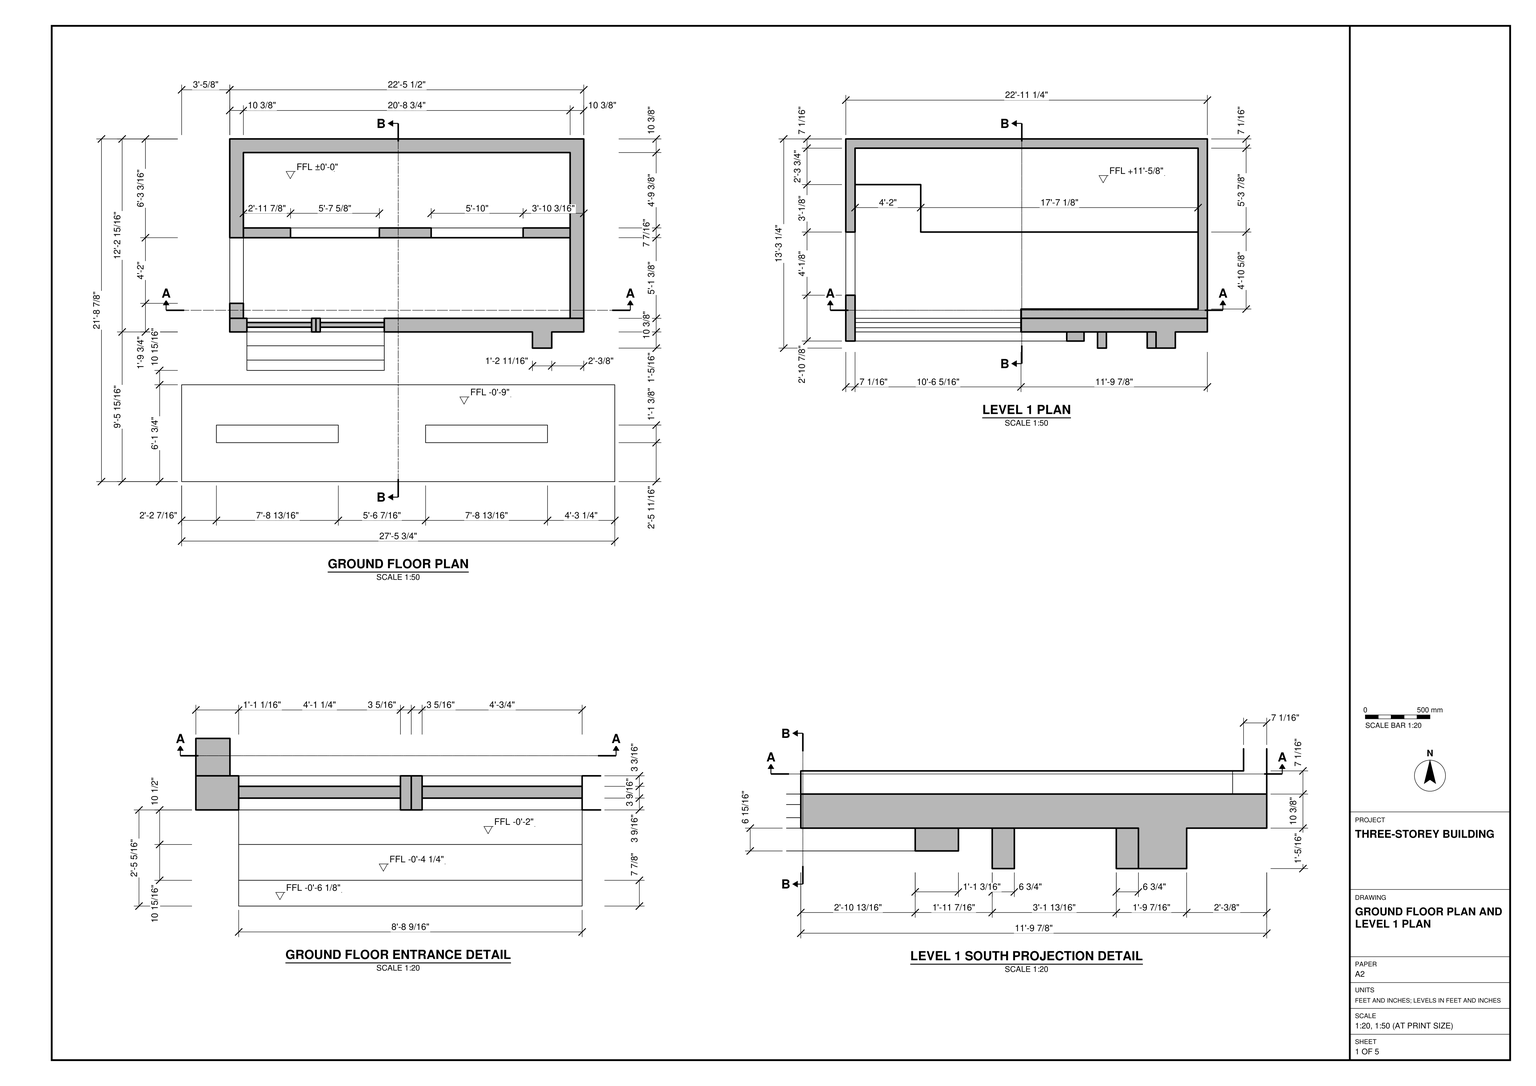
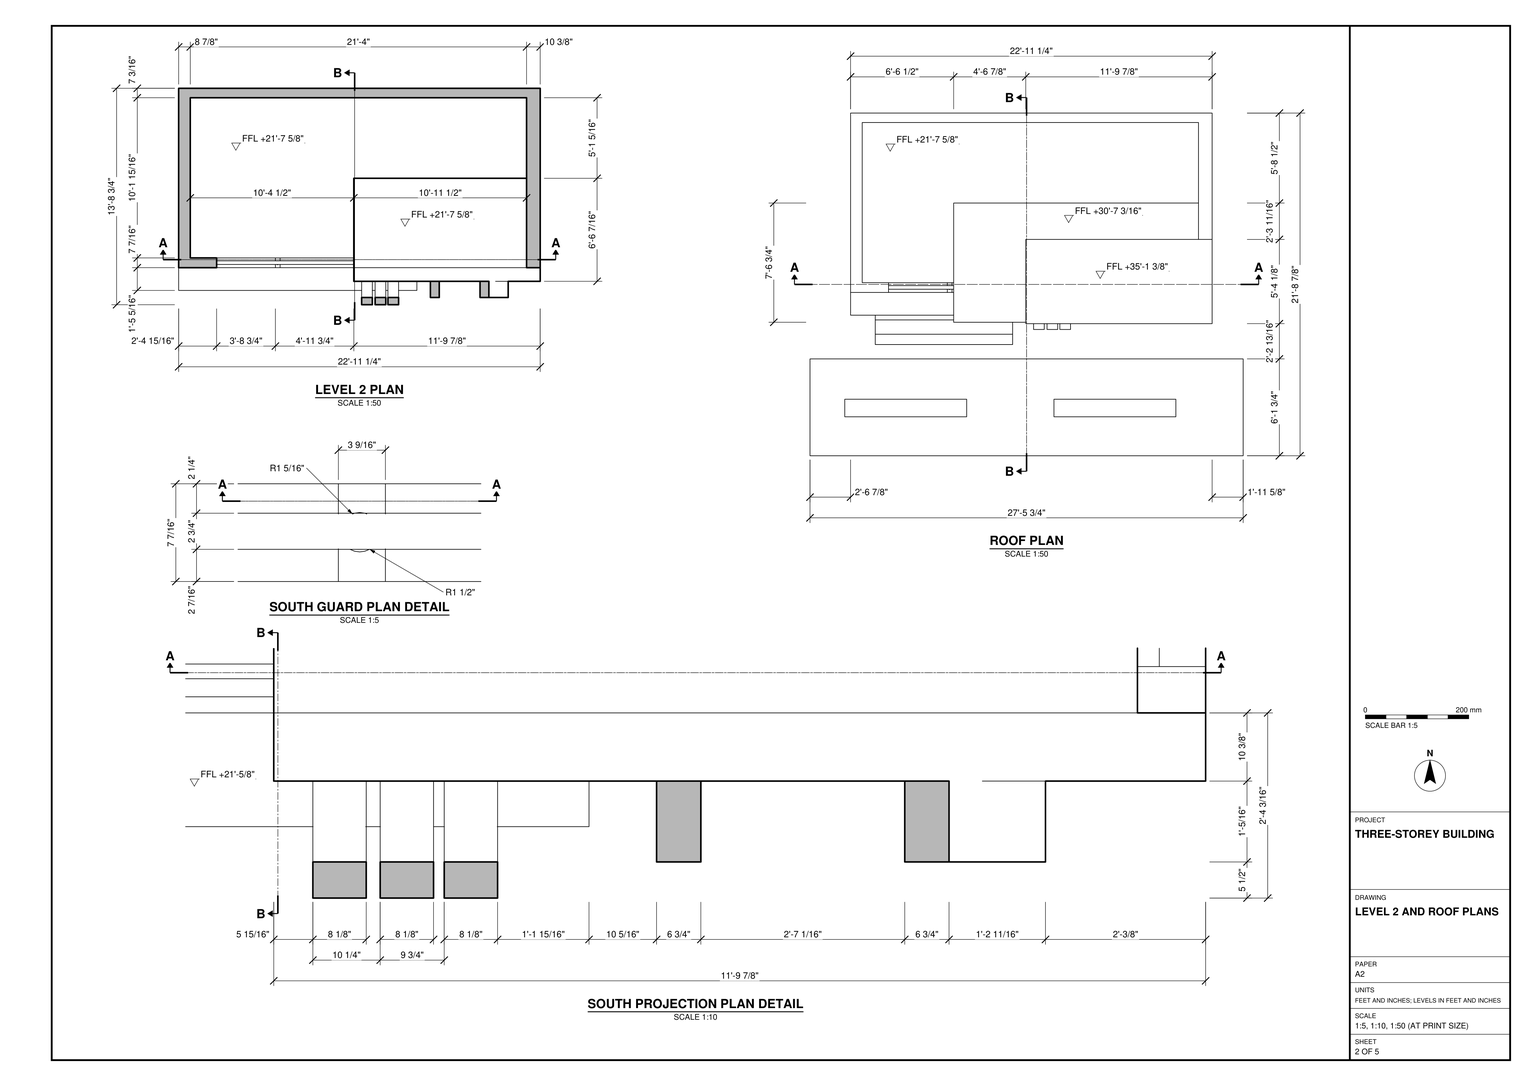
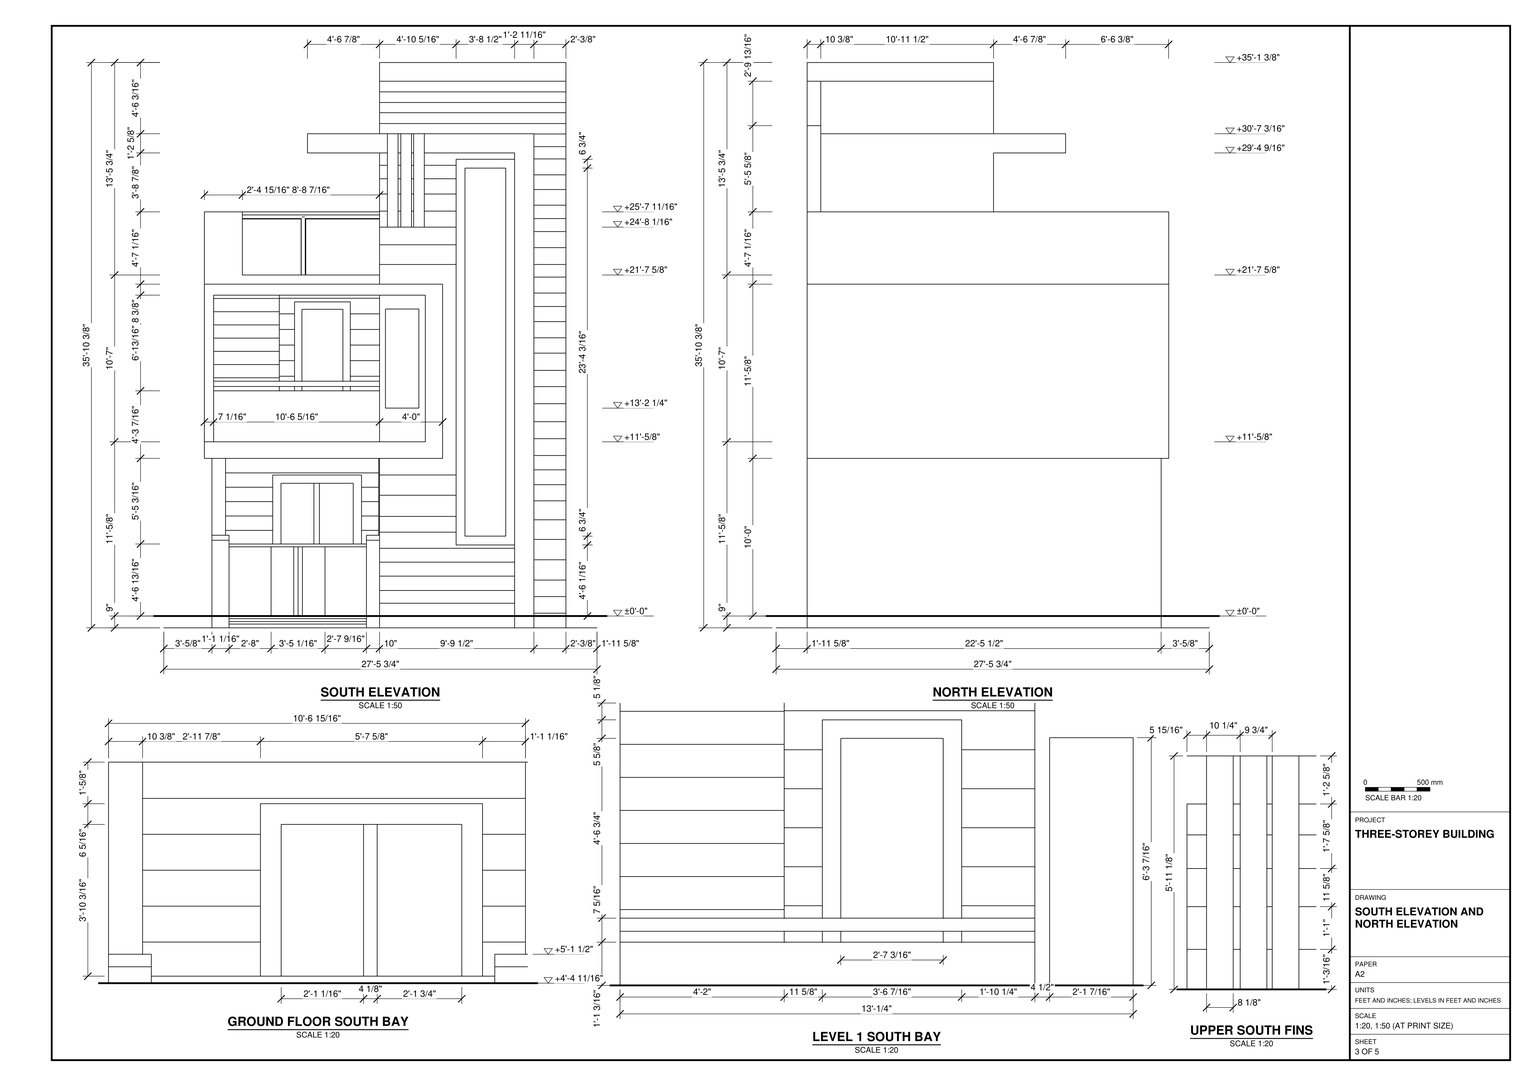
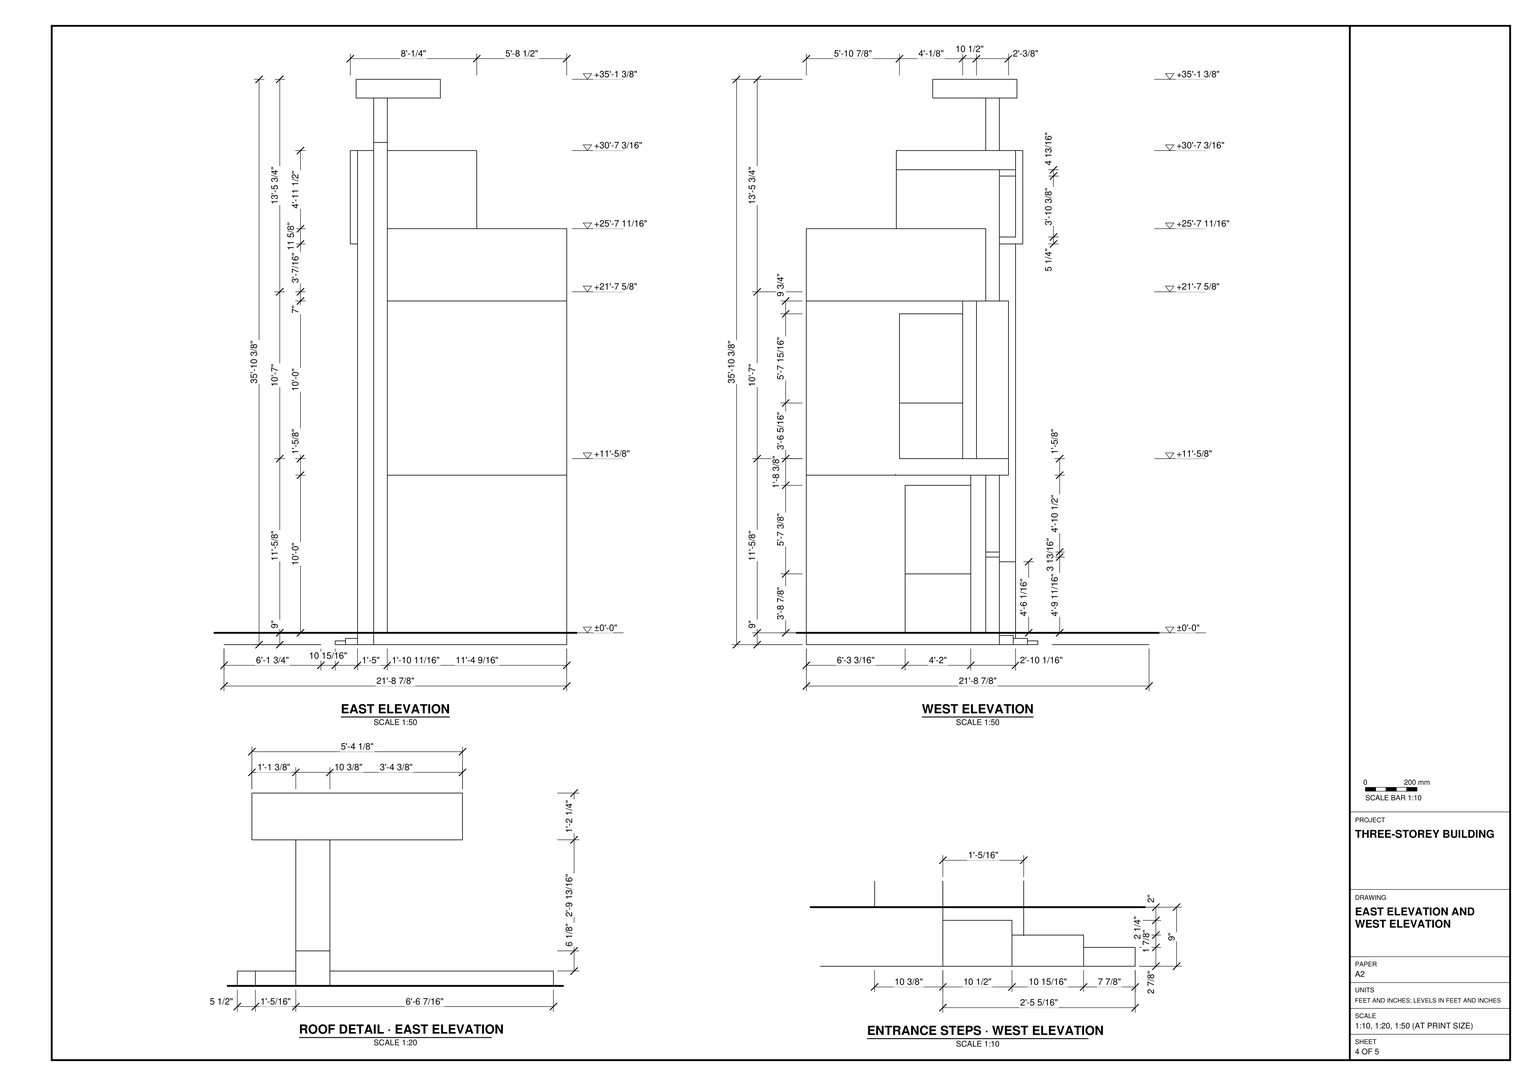
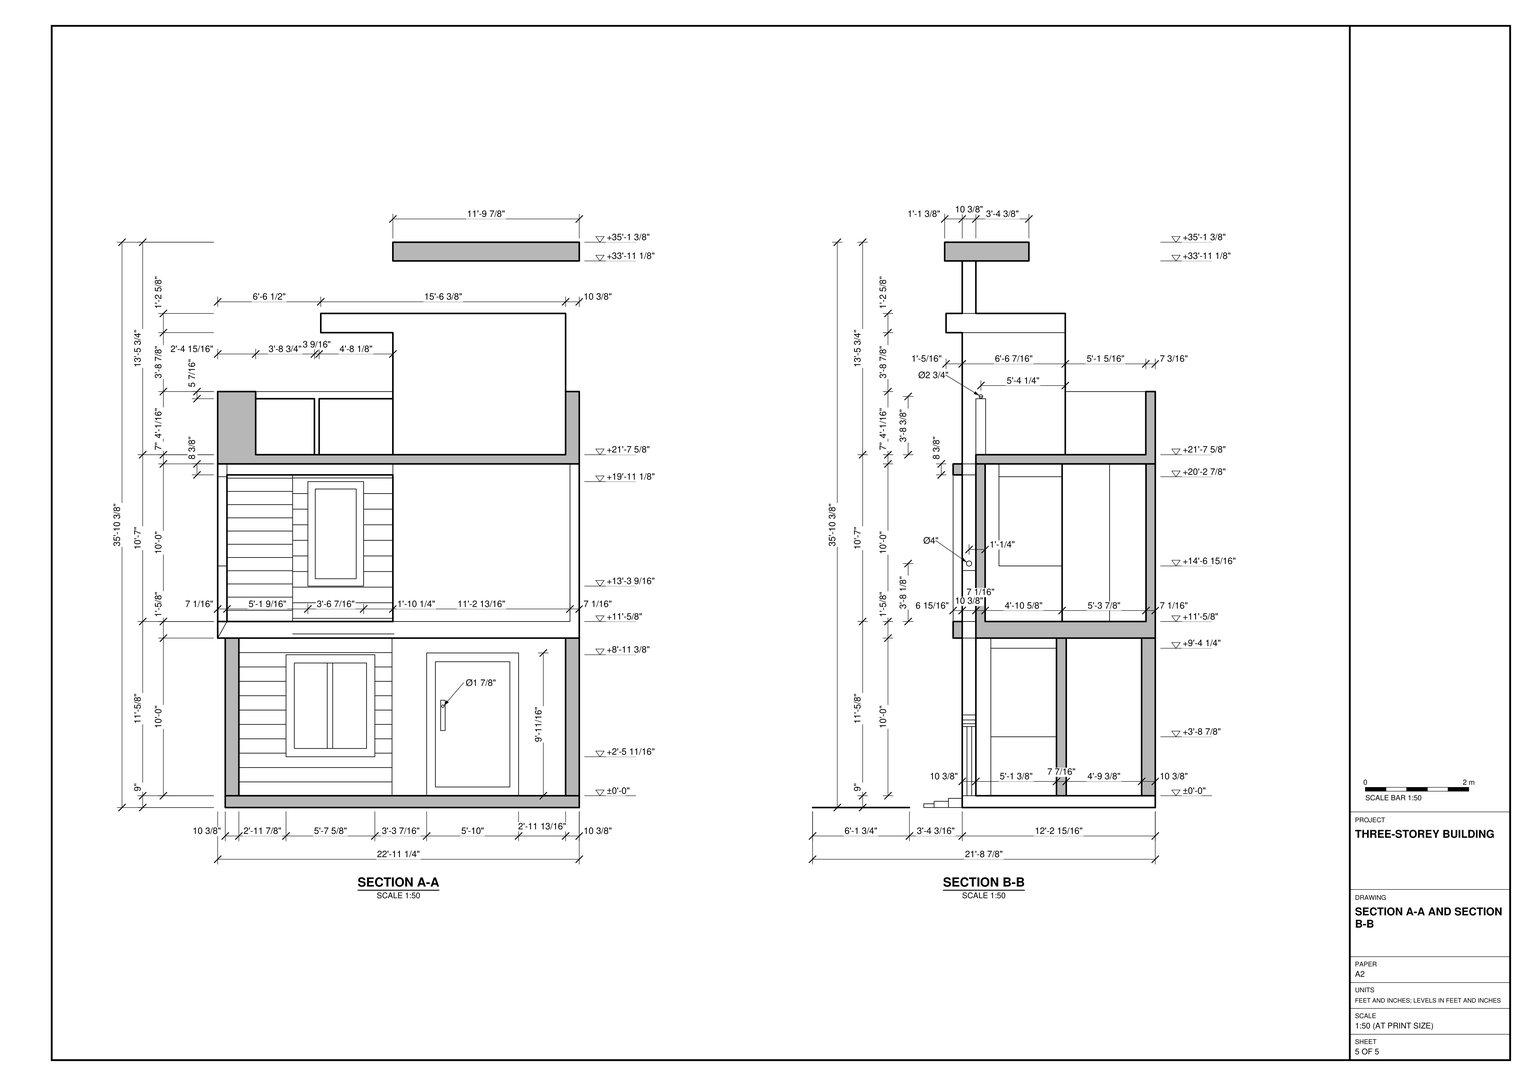
Build the three-storey building in SketchUp from task_files/diagram_01.pdf. Work in feet and inches. Set the ground floor at ±0'-0", Level 1 at +11'-5/8" and Level 2 at +21'-7 5/8". Including the ground strip in front of the entrance, the model must measure 27'-5 3/4" along X, 21'-8 7/8" along Y and 35'-10 3/8" along Z.

Follow the plan for each storey rather than repeating the ground-floor footprint. Model the floor slabs, walls and openings with the offsets and thicknesses drawn, including the 10 3/8" ground-floor side walls and the 7 1/16" Level 1 side walls. On the south side, build the entrance steps, the divided ground-floor opening and the projecting frame around the Level 1 bay. Use the enlarged details to place the guards, upper fins and tall framed panel. Match the horizontal divisions on the south face and the stepped outline of the flat roof to the elevations. Include the two narrow rectangular features on the front ground strip.

Keep walls, slabs and roof elements in separate groups or components. Keep each furniture or joinery piece shown separate, and use components for repeated parts. Any decor or loose items shown may be represented by suitable library components. Save one SketchUp model as output_files/three_storey_building_with_projecting_south_bays.skp.

# SketchUp Ruby script. Lengths in inches.
U = 1.inch
M = Sketchup.active_model
def pt(a) = Geom::Point3d.new(a.map { |v| v * U })
def face(e, loops, mat)
  f = e.add_face(loops[0].map { |a| pt(a) })
  loops[1..].each { |l| e.add_face(l.map { |a| pt(a) }).erase! }
  f.material = f.back_material = mat if mat
  f
end
# faces: each face lists its corners as indices into pts; further lists are holes
def faces(e, pts, list, mat = nil) = list.each { |f| face(e, (f[0].is_a?(Array) ? f : [f]).map { |l| l.map { |i| pts[i] } }, mat) }
# xy, xz, yz: faces in a plane at the given z, y or x. An outline is a flat list of corners, or four numbers for a rectangle; further outlines are holes
def ring(l) = l.size == 4 ? [[l[0], l[1]], [l[2], l[1]], [l[2], l[3]], [l[0], l[3]]] : l.each_slice(2).to_a
def flat(e, list, mat, &to3) = list.each { |f| face(e, (f[0].is_a?(Array) ? f : [f]).map { |l| ring(l).map { |u, v| to3.(u, v) } }, mat) }
def xy(e, z, list, mat = nil) = flat(e, list, mat) { |x, y| [x, y, z] }
def xz(e, y, list, mat = nil) = flat(e, list, mat) { |x, z| [x, y, z] }
def yz(e, x, list, mat = nil) = flat(e, list, mat) { |y, z| [x, y, z] }
def lines(e, pts, list) = list.each { |a, b| e.add_line(pt(pts[a]), pt(pts[b])) }
# prism: a flat outline (further loops are holes) pulled along v
def prism(e, loops, v, mat = nil)
  f = face(e, loops, mat); d = Geom::Vector3d.new(v.map { |x| x * U })
  f.pushpull(f.normal.samedirection?(d) ? d.length : -d.length)
end
def box(e, o, s, mat = nil) = prism(e, [[o, [o[0] + s[0], o[1], o[2]], [o[0] + s[0], o[1] + s[1], o[2]], [o[0], o[1] + s[1], o[2]]]], [0, 0, s[2]], mat)
def at(x, y, z, deg = 0) = Geom::Transformation.translation(pt([x, y, z])) * Geom::Transformation.rotation(ORIGIN, Z_AXIS, deg.degrees)
def axes(o, x, y, z) = Geom::Transformation.new([*x, 0, *y, 0, *z, 0, *pt(o).to_a, 1])
def part(name) = M.definitions.add(name)
# library, detail: a bought-in or finely detailed component or shape, given as its bounding box
def library(name, o, s) = part(name).tap { |d| box(d.entities, o, s) }
def detail(e, o, s) = box(e.add_group.entities, o, s)
def put(e, d, t, mat = nil) = e.add_instance(d, t).tap { |i| i.material = mat if mat }
def group(e, t, mat = nil) = e.add_group.tap { |g| g.transformation = t; g.material = mat if mat }.entities
root = M.entities
M.materials.add("[0012_Bisque]").color = [255, 228, 196]
M.materials.add("[0061_OliveDrab]").color = [96, 127, 31]
M.materials.add("[Asphalt New]").color = [67, 60, 62]
M.materials.add("[Carpet Diamond Yellow]").color = [226, 217, 124]
M.materials.add("[Color C01]").color = [255, 229, 204]
M.materials.add("[Color G02]").color = [104, 173, 104]
M.materials.add("[Concrete Aggregate Smoke]").color = [154, 150, 148]
M.materials.add("[Formica Beige]").color = [211, 187, 149]
M.materials.add("[Formica Graystone]").color = [149, 146, 135]
M.materials.add("[Formica Laminate Dark]").color = [50, 53, 60]
M.materials.add("[Formica Laminate Light]").color = [213, 189, 164]
M.materials.add("[Formica Speckled Grey]").color = [94, 105, 111]
M.materials.add("[Leather Blue]").color = [45, 57, 74]
M.materials.add("[Terrazzo Light Blue]").color = [196, 214, 227]
M.materials.add("[Terrazzo Tile Light]").color = [219, 217, 210]
M.materials.add("[Translucent Glass Blue]").color = [100, 149, 237]
M.materials["[Translucent Glass Blue]"].alpha = 0.5
M.materials.add("[Translucent Glass Safety]").color = [204, 235, 244]
M.materials["[Translucent Glass Safety]"].alpha = 0.5
M.materials.add("[Translucent Glass Sky Reflection]").color = [126, 138, 183]
M.materials["[Translucent Glass Sky Reflection]"].alpha = 0.52
M.materials.add("[Wood Bamboo]").color = [177, 105, 43]
M.materials.add("[Wood Cherry Original]").color = [152, 86, 42]
M.materials.add("[Wood Floor Light]").color = [204, 176, 127]
M.materials.add("[Wood Veneer 01]").color = [120, 70, 37]
xy(root,0,[[49.68,84.67,154.26,92.52],[49.68,92.52,154.26,103.43],[267.0625,101.64,281.74,113.95],[49.68,103.43,154.26,113.95],[36.64,113.95,306.13,260.9]])
xy(root,0,[[[0,0,329.75,73.75],[26.46,29.67,119.27,43.05],[185.71,29.67,278.52,43.05]]],"[Formica Graystone]")
xy(root,0,[[26.46,29.67,119.27,43.05],[185.71,29.67,278.52,43.05]],"[Formica Laminate Dark]")
xy(root,2.875,[[49.68,84.67,154.26,92.52]],"[Terrazzo Light Blue]")
xy(root,4.75,[[49.68,92.52,154.26,103.43]],"[Terrazzo Light Blue]")
xy(root,6.99,[[49.68,103.43,154.26,113.95]],"[Terrazzo Light Blue]")
xy(root,9,[[98.93,113.95,102.23,124.33],[102.23,113.95,105.53,124.33],[49.68,117.54,98.93,121.14],[105.53,117.54,154.26,121.14],[295.75,124.33,295.75,250.52,47.02,250.52,47.02,185.7,36.64,185.7,36.64,260.9,306.13,260.9,306.13,124.33],
  [36.64,124.33,47.02,135.73],[36.64,135.73,47.02,185.7],[47.02,185.7,189.96,193.125],[189.96,185.7,259.96,193.125],[259.96,185.7,295.75,193.125],
  [47.02,193.125,295.75,250.52]])
xy(root,9,[[49.68,113.95,98.93,117.54],[105.53,113.95,154.26,117.54]],"[Asphalt New]")
xy(root,9,[[49.68,121.14,98.93,124.33],[105.53,121.14,154.26,124.33]],"[Formica Laminate Dark]")
xy(root,9,[[47.02,124.33,295.75,185.7]],"[Leather Blue]")
xy(root,38.66,[[82.9,185.7,150.52,193.125]])
xy(root,53.875,[[36.64,135.73,47.02,185.7]],"[Terrazzo Tile Light]")
xy(root,61.69,[[98.93,113.95,102.23,117.54],[102.23,113.95,105.53,117.54],[49.68,117.54,98.93,121.14],[98.93,117.54,102.23,121.14],[102.23,117.54,105.53,121.14],
  [105.53,117.54,154.26,121.14],[49.68,121.14,98.93,124.33],[98.93,121.14,102.23,124.33],[102.23,121.14,105.53,124.33],[105.53,121.14,154.26,124.33]])
xy(root,61.69,[[49.68,113.95,98.93,117.54],[105.53,113.95,154.26,117.54]],"[Asphalt New]")
xy(root,63.08,[[222.54,101.64,267.0625,113.95]])
xy(root,63.83,[[49.68,113.95,154.26,124.33]],"[Asphalt New]")
xy(root,66.6875,[[36.64,113.95,49.68,124.33],[154.26,113.95,164.25,124.33]])
xy(root,69.82,[[229.28,101.64,260.32,113.95]])
xy(root,70.5,[[36.64,113.95,49.68,124.33],[154.26,113.95,164.25,124.33]])
xy(root,116.35,[[82.9,185.7,150.52,193.125]])
xy(root,117.6875,[[189.96,185.7,259.96,193.125]])
xy(root,121.28,[[36.64,135.73,47.02,185.7]])
xy(root,129,[[30.89,107.01,36.64,135.73],[36.64,107.01,47.02,124.33],[47.02,107.01,47.02,185.7,295.75,185.7,295.75,124.33,164.25,124.33,164.25,113.95,212.25,113.95,212.25,107.01],[36.64,124.33,47.02,135.73],[295.75,124.33,306.13,185.7],
  [30.89,135.73,36.64,185.7],[36.64,135.73,47.02,185.7],[30.89,185.7,36.64,193.125],[36.64,185.7,47.02,193.125],[47.02,185.7,295.75,193.125],
  [295.75,185.7,306.13,193.125],[30.89,193.125,36.64,260.9],[36.64,193.125,47.02,260.9],[47.02,193.125,295.75,250.52],[295.75,193.125,306.13,260.9],
  [47.02,250.52,295.75,260.9]])
xy(root,141.625,[[30.89,107.01,37.94,131.39],[37.94,107.01,199.09,113.95],[37.94,113.95,164.25,124.33],[30.89,131.39,37.94,141.9],[30.89,141.9,37.94,190],
  [87.93,190,299.07,190,299.07,253.85,37.94,253.85,37.94,226.125,87.93,226.125]])
xy(root,141.625,[[30.89,107.01,30.89,131.39,37.94,131.39,37.94,124.33,164.25,124.33,164.25,131.39,299.07,131.39,299.07,190,87.93,190,87.93,226.125,37.94,226.125,37.94,107.01]],"[Carpet Diamond Yellow]")
xy(root,180.4375,[[37.94,113.95,164.25,124.33]],"[Translucent Glass Safety]")
xy(root,183.9375,[[30.89,141.9,37.94,190]],"[Terrazzo Tile Light]")
xy(root,251.87,[[30.89,141.9,37.94,190]])
xy(root,253.26,[[37.94,107.01,37.94,131.39,164.25,131.39,164.25,113.95,199.09,113.95,199.09,107.01]])
xy(root,261.625,[[30.89,107.01,212.25,107.01,212.25,113.95,164.25,113.95,164.25,124.33,30.89,124.33],[30.89,124.33,164.25,131.39],[164.25,124.33,306.13,131.39],[30.89,131.39,37.94,141.9],[37.94,131.39,37.94,226.125,87.93,226.125,87.93,190,299.07,190,299.07,131.39],
  [299.07,131.39,306.13,190],[30.89,141.9,37.94,226.125],[87.93,190,87.93,226.125,37.94,226.125,37.94,253.85,299.07,253.85,299.07,190],[299.07,190,306.13,253.85],[30.89,226.125,37.94,260.9],
  [37.94,253.85,306.13,260.9]])
xy(root,268.625,[[59.81,124.33,104.53,131.77],[[104.53,124.33,108.11,131.77],[106.16,126.59,105.77,126.64,105.41,126.79,105.09,127.03,104.86,127.34,104.71,127.7,104.66,128.09,104.71,128.48,104.86,128.84,105.09,129.15,105.41,129.39,105.77,129.54,106.16,129.59,106.54,129.54,106.91,129.39,107.22,129.15,107.45,128.84,107.6,128.48,107.66,128.09,107.6,127.7,107.45,127.34,107.22,127.03,106.91,126.79,106.54,126.64]],[108.11,124.33,164.25,131.77],[164.25,124.33,295.75,192.4],[106.16,126.59,105.77,126.64,105.41,126.79,105.09,127.03,104.86,127.34,104.71,127.7,104.66,128.09,104.71,128.48,104.86,128.84,105.09,129.15,105.41,129.39,105.77,129.54,106.16,129.59,106.54,129.54,106.91,129.39,107.22,129.15,107.45,128.84,107.6,128.48,107.66,128.09,107.6,127.7,107.45,127.34,107.22,127.03,106.91,126.79,106.54,126.64],
  [39.75,131.77,164.25,131.77,164.25,192.4,295.75,192.4,295.75,253.71,39.75,253.71]])
xy(root,305.07,[[170.2,96.14,178.33,113.95],[180.45,96.14,188.58,113.95],[190.2,96.14,198.33,113.95]],"[Formica Speckled Grey]")
xy(root,310.32,[[170.2,101.64,178.33,113.95],[180.45,101.64,188.58,113.95],[190.2,101.64,198.33,113.95]],"[Formica Speckled Grey]")
xy(root,311.25,[[59.81,124.33,104.53,131.77],[108.11,124.33,164.25,131.77]],"[Translucent Glass Safety]")
xy(root,312.8125,[[106.16,126.59,106.54,126.64,106.91,126.79,107.22,127.03,107.45,127.34,107.6,127.7,107.66,128.09,107.6,128.48,107.45,128.84,107.22,129.15,106.91,129.39,106.54,129.54,106.16,129.59,105.77,129.54,105.41,129.39,105.09,129.15,104.86,128.84,104.71,128.48,104.66,128.09,104.71,127.7,104.86,127.34,105.09,127.03,105.41,126.79,105.77,126.64]])
xy(root,316.6875,[[30.89,124.33,59.81,124.33,59.81,131.77,39.75,131.77,39.75,253.71,295.75,253.71,295.75,124.33,306.13,124.33,306.13,260.9,30.89,260.9]],"[Formica Graystone]")
xy(root,349.99,[[229.28,101.64,260.32,113.95]])
xy(root,356.73,[[222.54,101.64,267.0625,113.95]])
xy(root,361.53,[[109.375,101.64,109.375,192.4,164.25,192.4,164.25,113.95,267.0625,113.95,267.0625,101.64]],"[0012_Bisque]")
xy(root,376.17,[[109.375,101.64,281.74,101.64,281.74,113.95,164.25,113.95,164.25,124.33,295.75,124.33,295.75,192.4,109.375,192.4]])
xy(root,376.17,[[170.2,96.14,178.33,101.64],[180.45,96.14,188.58,101.64],[190.2,96.14,198.33,101.64]],"[Formica Speckled Grey]")
xy(root,416.125,[[164.25,100.58,306.13,113.95],[164.25,113.95,306.13,124.33],[164.25,124.33,295.75,164.71],[295.75,124.33,306.13,164.71]])
xy(root,430.375,[[164.25,100.58,306.13,164.71]])
xz(root,84.67,[[49.68,0,154.26,2.875]],"[Terrazzo Light Blue]")
xz(root,92.52,[[49.68,0,154.26,2.875]])
xz(root,92.52,[[49.68,2.875,154.26,4.75]],"[Terrazzo Light Blue]")
xz(root,96.14,[[170.2,305.07,178.33,376.17],[180.45,305.07,188.58,376.17],[190.2,305.07,198.33,376.17]],"[Formica Speckled Grey]")
xz(root,100.58,[[164.25,416.125,306.13,430.375]])
xz(root,101.64,[[267.0625,0,281.74,0,281.74,376.17,198.33,376.17,198.33,361.53,267.0625,361.53],[[222.54,63.08,267.0625,356.73],[229.28,69.82,260.32,349.99]],[109.375,361.53,170.2,376.17],[170.2,361.53,178.33,376.17],[178.33,361.53,180.45,376.17],
  [180.45,361.53,188.58,376.17],[188.58,361.53,190.2,376.17],[190.2,361.53,198.33,376.17]])
xz(root,101.64,[[170.2,310.32,178.33,361.53],[180.45,310.32,188.58,361.53],[190.2,310.32,198.33,361.53]],"[Formica Speckled Grey]")
xz(root,103.43,[[49.68,0,154.26,4.75]])
xz(root,103.43,[[49.68,4.75,154.26,6.99]],"[Terrazzo Light Blue]")
xz(root,107.01,[[30.89,129,212.25,129,212.25,261.625,30.89,261.625,30.89,141.625,37.94,141.625,37.94,253.26,199.09,253.26,199.09,141.625,30.89,141.625]])
xz(root,113.95,[[49.68,0,154.26,6.99],[[222.54,63.08,267.0625,356.73],[229.28,69.82,260.32,349.99]],[36.64,66.6875,49.68,70.5],[154.26,66.6875,164.25,70.5],[164.25,129,212.25,129,212.25,253.26,199.09,253.26,199.09,141.625,164.25,141.625],
  [164.25,253.26,212.25,261.625],[170.2,305.07,178.33,310.32],[180.45,305.07,188.58,310.32]])
xz(root,113.95,[[49.68,6.99,154.26,9],[98.93,9,102.23,61.69],[102.23,9,105.53,61.69],[49.68,61.69,154.26,63.83]],"[Asphalt New]")
xz(root,113.95,[[36.64,0,49.68,66.6875],[154.26,0,164.25,66.6875],[164.25,0,267.0625,9],[281.74,0,306.13,11.125],[164.25,9,267.0625,18.71],
  [281.74,11.125,306.13,23.8125],[164.25,18.71,267.0625,28.43],[281.74,23.8125,306.13,36.375],[164.25,28.43,267.0625,39.37],[281.74,36.375,306.13,51.8125],
  [164.25,39.37,267.0625,49.99],[164.25,49.99,267.0625,60.55],[281.74,51.8125,306.13,67.3125],[164.25,60.55,267.0625,60.55,267.0625,63.08,222.54,63.08,222.54,72.82,164.25,72.82],[281.74,67.3125,306.13,82.25],
  [164.25,72.82,222.54,84.82],[281.74,82.25,306.13,96.6875],[164.25,84.82,222.54,100.94],[281.74,96.6875,306.13,109],[164.25,100.94,222.54,116.38],
  [281.74,109,306.13,120.3125],[164.25,116.38,222.54,116.38,222.54,276.625,164.25,276.625,164.25,261.625,212.25,261.625,212.25,129,164.25,129],[281.74,120.3125,306.13,131.1875],[281.74,131.1875,306.13,144],[[164.25,141.625,199.09,253.26],[168.75,167.27,194.18,242.71]],
  [281.74,144,306.13,156.9375],[281.74,156.9375,306.13,170.625],[281.74,170.625,306.13,183.625],[281.74,183.625,306.13,196],[281.74,196,306.13,209.125],
  [281.74,209.125,306.13,220.8125],[281.74,220.8125,306.13,233.125],[281.74,233.125,306.13,244.625],[281.74,244.625,306.13,254.875],[281.74,254.875,306.13,267],
  [281.74,267,306.13,276.625],[164.25,276.625,222.54,291.63],[281.74,276.625,306.13,289.4375],[281.74,289.4375,306.13,301.6875],[164.25,291.63,222.54,305.07],
  [281.74,301.6875,306.13,311.5625],[164.25,305.07,170.2,305.07,170.2,310.32,178.33,310.32,178.33,305.07,180.45,305.07,180.45,310.32,188.58,310.32,188.58,305.07,190.2,305.07,190.2,310.32,198.33,310.32,198.33,305.07,222.54,305.07,222.54,317.25,164.25,317.25],[281.74,311.5625,306.13,321.75],[164.25,317.25,222.54,330.26],[281.74,321.75,306.13,333.6875],
  [164.25,330.26,222.54,341.88],[281.74,333.6875,306.13,344.875],[164.25,341.88,222.54,352.12],[281.74,344.875,306.13,357],[164.25,352.12,222.54,352.12,222.54,356.73,267.0625,356.73,267.0625,361.53,164.25,361.53],
  [281.74,357,306.13,366.34],[281.74,366.34,306.13,375.97],[281.74,375.97,306.13,375.97,306.13,383.92,164.25,383.92,164.25,376.17,281.74,376.17],[164.25,383.92,306.13,392.17],[164.25,392.17,306.13,399.92],
  [164.25,399.92,306.13,408.02],[164.25,408.02,306.13,416.125]],"[Color G02]")
xz(root,113.95,[[168.75,167.27,194.18,242.71]],"[Concrete Aggregate Smoke]")
xz(root,113.95,[[37.94,141.625,164.25,180.4375]],"[Translucent Glass Safety]")
xz(root,113.95,[[229.28,69.82,260.32,349.99]],"[Translucent Glass Sky Reflection]")
xz(root,117.54,[[81.68,9,98.93,61.69],[105.53,9,122.73,61.69]],"[Concrete Aggregate Smoke]")
xz(root,117.54,[[49.68,9,81.68,61.69],[122.73,9,154.26,61.69]],"[Wood Bamboo]")
xz(root,121.14,[[49.68,9,98.93,61.69],[105.53,9,154.26,61.69]],"[Formica Laminate Dark]")
xz(root,124.33,[[36.64,9,47.02,66.6875],[47.02,9,49.68,66.6875],[164.25,9,295.75,129],[295.75,9,306.13,129],[36.64,66.6875,47.02,70.5],
  [47.02,66.6875,49.68,70.5],[154.26,66.6875,164.25,70.5],[164.25,129,295.75,261.625],[295.75,129,306.13,261.625],[164.25,261.625,295.75,268.625],
  [295.75,261.625,306.13,316.6875],[295.75,316.6875,306.13,382.3125],[164.25,376.17,295.75,416.125],[295.75,382.3125,306.13,416.125]])
xz(root,124.33,[[30.89,261.625,164.25,261.625,164.25,268.625,59.81,268.625,59.81,316.6875,30.89,316.6875]],"[0061_OliveDrab]")
xz(root,124.33,[[98.93,9,102.23,61.69],[102.23,9,105.53,61.69],[154.26,9,164.25,66.6875],[49.68,61.69,154.26,63.83]],"[Asphalt New]")
xz(root,124.33,[[36.64,70.5,47.02,129]],"[Terrazzo Tile Light]")
xz(root,124.33,[[37.94,141.625,164.25,180.4375],[59.81,268.625,104.53,311.25],[108.11,268.625,164.25,311.25]],"[Translucent Glass Safety]")
xz(root,131.39,[[164.25,141.625,299.07,261.625],[37.94,253.26,164.25,261.625]])
xz(root,131.77,[[39.75,268.625,59.81,316.6875]],"[Color C01]")
xz(root,131.77,[[59.81,268.625,104.53,311.25],[108.11,268.625,164.25,311.25]],"[Translucent Glass Safety]")
xz(root,135.73,[[36.64,9,47.02,53.875]])
xz(root,135.73,[[36.64,53.875,47.02,121.28]],"[Terrazzo Tile Light]")
xz(root,141.9,[[30.89,183.9375,37.94,251.87]])
xz(root,164.71,[[164.25,416.125,306.13,430.375]])
xz(root,185.7,[[36.64,9,47.02,53.875]])
xz(root,185.7,[[47.02,9,163.6,19.52],[163.6,9,189.96,9,189.96,117.6875,259.96,117.6875,259.96,9,295.75,9,295.75,129,163.6,129],[47.02,19.52,163.6,30.46],[47.02,30.46,163.6,30.46,163.6,41.4,150.52,41.4,150.52,38.66,82.9,38.66,82.9,41.4,47.02,41.4],[47.02,41.4,82.9,52.33],
  [150.52,41.4,163.6,52.33],[47.02,52.33,82.9,63.27],[150.52,52.33,163.6,63.27],[47.02,63.27,82.9,74.21],[150.52,63.27,163.6,74.21],
  [47.02,74.21,82.9,85.15],[150.52,74.21,163.6,85.15],[47.02,85.15,82.9,96.08],[150.52,85.15,163.6,96.08],[47.02,96.08,82.9,107.02],
  [150.52,96.08,163.6,107.02],[47.02,107.02,82.9,107.02,82.9,116.35,150.52,116.35,150.52,107.02,163.6,107.02,163.6,117.96,47.02,117.96],[47.02,117.96,163.6,129]],"[Color G02]")
xz(root,185.7,[[202.26,76.21,202.5,76.25,202.72,76.34,202.92,76.49,203.07,76.68,203.16,76.91,203.19,77.15,203.16,77.39,203.07,77.62,202.92,77.81,202.72,77.96,202.5,78.06,202.26,78.09,202.01,78.06,201.79,77.96,201.59,77.81,201.44,77.62,201.35,77.39,201.32,77.15,201.35,76.91,201.44,76.68,201.59,76.49,201.79,76.34,202.01,76.25]],"[Formica Beige]")
xz(root,185.7,[[[189.96,9,259.96,117.6875],[196.61,15.65,253.3,111.04]]],"[Formica Graystone]")
xz(root,185.7,[[[82.9,38.66,150.52,116.35],[89.21,44.98,144.21,110.04]],[114.29,44.98,118.45,110.04],[[200.625,58.61,204.0625,81.67],[202.26,76.21,202.01,76.25,201.79,76.34,201.59,76.49,201.44,76.68,201.35,76.91,201.32,77.15,201.35,77.39,201.44,77.62,201.59,77.81,201.79,77.96,202.01,78.06,202.26,78.09,202.5,78.06,202.72,77.96,202.92,77.81,203.07,77.62,203.16,77.39,203.19,77.15,203.16,76.91,203.07,76.68,202.92,76.49,202.72,76.34,202.5,76.25]]],"[Formica Laminate Dark]")
xz(root,185.7,[[[196.61,15.65,253.3,111.04],[200.625,58.61,204.0625,81.67]]],"[Formica Laminate Light]")
xz(root,185.7,[[36.64,53.875,47.02,121.28]],"[Terrazzo Tile Light]")
xz(root,185.7,[[89.21,44.98,114.29,110.04],[118.45,44.98,144.21,110.04]],"[Translucent Glass Blue]")
xz(root,190,[[87.93,141.625,165.2,144.04],[165.2,141.625,222.58,141.625,222.58,250.125,279.39,250.125,279.39,141.625,299.07,141.625,299.07,261.625,165.2,261.625],[87.93,144.04,165.2,155.91],[87.93,155.91,165.2,167.79],[87.93,167.79,165.2,167.79,165.2,179.66,141.97,179.66,141.97,168.57,99.53,168.57,99.53,179.66,87.93,179.66],
  [87.93,179.66,99.53,191.54],[141.97,179.66,165.2,191.54],[87.93,191.54,99.53,203.41],[141.97,191.54,165.2,203.41],[87.93,203.41,99.53,215.29],
  [141.97,203.41,165.2,215.29],[87.93,215.29,99.53,227.16],[141.97,215.29,165.2,227.16],[87.93,227.16,99.53,239.04],[141.97,227.16,165.2,239.04],
  [87.93,239.04,99.53,239.04,99.53,248.13,141.97,248.13,141.97,239.04,165.2,239.04,165.2,250.91,87.93,250.91],[87.93,250.91,165.2,261.625]],"[Color G02]")
xz(root,190,[[99.53,168.57,141.97,168.57,141.97,179.66,136.34,179.66,136.34,174.2,105.16,174.2,105.16,242.5,136.34,242.5,136.34,239.04,141.97,239.04,141.97,248.13,99.53,248.13],[136.34,179.66,141.97,191.54],[136.34,191.54,141.97,203.41],[136.34,203.41,141.97,215.29],[136.34,215.29,141.97,227.16],
  [136.34,227.16,141.97,239.04]],"[Formica Laminate Dark]")
xz(root,190,[[30.89,183.9375,37.94,251.87]],"[Terrazzo Tile Light]")
xz(root,190,[[105.16,174.2,136.34,242.5]],"[Translucent Glass Safety]")
xz(root,190,[[[230.01,149.05,271.97,242.7],[233.75,187.8125,237.375,215.5]]],"[Wood Cherry Original]")
xz(root,190,[[233.75,187.8125,237.375,215.5]],"[Wood Floor Light]")
xz(root,190,[[[222.58,141.625,279.39,250.125],[230.01,149.05,271.97,242.7]]],"[Wood Veneer 01]")
xz(root,192.4,[[164.25,268.625,164.25,361.53,109.375,361.53,109.375,376.17,295.75,376.17,295.75,268.625]],"[0012_Bisque]")
xz(root,193.125,[[[47.02,9,47.02,129,295.75,129,295.75,9,259.96,9,259.96,117.6875,189.96,117.6875,189.96,9],[82.9,38.66,150.52,116.35]]])
xz(root,226.125,[[37.94,141.625,87.93,150.11],[37.94,150.11,87.93,160.18],[37.94,160.18,87.93,170.24],[37.94,170.24,87.93,180.3],[37.94,180.3,87.93,190.36],
  [37.94,190.36,87.93,200.43],[37.94,200.43,87.93,210.49],[37.94,210.49,87.93,220.55],[37.94,220.55,87.93,230.61],[37.94,230.61,87.93,240.68],
  [37.94,240.68,87.93,250.74],[37.94,250.74,87.93,261.625]],"[Color G02]")
xz(root,250.52,[[47.02,9,295.75,129]])
xz(root,253.71,[[39.75,268.625,295.75,316.6875]],"[Color C01]")
xz(root,253.85,[[37.94,141.625,299.07,261.625]])
xz(root,260.9,[[36.64,0,306.13,9],[36.64,9,306.13,129],[30.89,129,306.13,261.625]],"[0012_Bisque]")
xz(root,260.9,[[30.89,261.625,306.13,316.6875]],"[0061_OliveDrab]")
yz(root,30.89,[[107.01,141.625,131.39,261.625]])
yz(root,30.89,[[124.33,261.625,260.9,316.6875]],"[0061_OliveDrab]")
yz(root,30.89,[[107.01,129,107.01,141.625,190,141.625,190,251.87,141.9,251.87,141.9,261.625,260.9,261.625,260.9,129],[131.39,141.625,141.9,261.625],[141.9,141.625,190,183.9375]],"[Terrazzo Tile Light]")
yz(root,36.64,[[113.95,66.6875,124.33,70.5]])
yz(root,36.64,[[113.95,0,113.95,66.6875,124.33,66.6875,124.33,9,260.9,9,260.9,0]],"[Color G02]")
yz(root,36.64,[[124.33,9,135.73,129],[135.73,9,185.7,53.875],[185.7,9,185.7,121.28,135.73,121.28,135.73,129,260.9,129,260.9,9]],"[Terrazzo Tile Light]")
yz(root,37.94,[[[107.01,141.625,113.95,141.625,113.95,180.4375,124.33,180.4375,124.33,141.625,131.39,141.625,131.39,253.26,107.01,253.26],[119.14,183.75,118.625,183.82,118.14,184.02,117.73,184.34,117.41,184.75,117.21,185.24,117.14,185.75,117.21,186.27,117.41,186.75,117.73,187.17,118.14,187.49,118.625,187.6875,119.14,187.75,119.66,187.6875,120.14,187.49,120.56,187.17,120.875,186.75,121.07,186.27,121.14,185.75,121.07,185.24,120.875,184.75,120.56,184.34,120.14,184.02,119.66,183.82]],[113.95,141.625,124.33,180.4375],[226.125,141.625,253.85,261.625]])
yz(root,37.94,[[131.39,141.625,226.125,141.625,226.125,261.625,141.9,261.625,141.9,251.87,190,251.87,190,183.9375,141.9,183.9375,141.9,261.625,131.39,261.625]],"[Terrazzo Tile Light]")
yz(root,39.75,[[131.77,268.625,253.71,316.6875]],"[Color C01]")
yz(root,47.02,[[185.7,9,193.125,129],[193.125,9,250.52,129],[135.73,121.28,185.7,129]])
yz(root,47.02,[[124.33,9,135.73,129],[135.73,9,185.7,53.875]],"[Terrazzo Tile Light]")
yz(root,49.68,[[117.54,9,121.14,61.69],[121.14,9,124.33,61.69],[113.95,61.69,124.33,63.83],[113.95,66.6875,124.33,70.5]])
yz(root,49.68,[[113.95,9,117.54,61.69],[113.95,63.83,124.33,66.6875]],"[Color G02]")
yz(root,49.68,[[84.67,0,92.52,2.875],[92.52,0,103.43,4.75],[103.43,0,113.95,6.99]],"[Terrazzo Light Blue]")
yz(root,59.81,[[124.33,268.625,131.77,311.25],[[124.33,311.25,131.77,316.6875],[128.16,311.6,127.8,311.65,127.47,311.78,127.1875,312,126.97,312.29,126.83,312.62,126.78,312.97,126.83,313.33,126.97,313.66,127.1875,313.95,127.47,314.17,127.8,314.3,128.16,314.35,128.51,314.3,128.85,314.17,129.13,313.95,129.35,313.66,129.49,313.33,129.53,312.97,129.49,312.62,129.35,312.29,129.13,312,128.85,311.78,128.51,311.65]],[128.16,311.6,127.8,311.65,127.47,311.78,127.1875,312,126.97,312.29,126.83,312.62,126.78,312.97,126.83,313.33,126.97,313.66,127.1875,313.95,127.47,314.17,127.8,314.3,128.16,314.35,128.51,314.3,128.85,314.17,129.13,313.95,129.35,313.66,129.49,313.33,129.53,312.97,129.49,312.62,129.35,312.29,129.13,312,128.85,311.78,128.51,311.65]])
yz(root,82.9,[[185.7,38.66,193.125,116.35]])
yz(root,87.93,[[190,141.625,226.125,261.625]],"[Color G02]")
yz(root,98.93,[[117.54,9,121.14,61.69]])
yz(root,98.93,[[113.95,9,117.54,61.69],[121.14,9,124.33,61.69]],"[Asphalt New]")
yz(root,102.23,[[113.95,9,124.33,61.69]])
yz(root,104.53,[[124.33,268.625,131.77,311.25]])
yz(root,105.53,[[117.54,9,121.14,61.69]])
yz(root,105.53,[[113.95,9,117.54,61.69]],"[Asphalt New]")
yz(root,105.53,[[121.14,9,124.33,61.69]],"[Formica Laminate Dark]")
yz(root,108.11,[[124.33,268.625,131.77,311.25]])
yz(root,109.375,[[101.64,361.53,192.4,376.17]])
yz(root,150.52,[[185.7,38.66,193.125,116.35]])
yz(root,154.26,[[117.54,9,121.14,61.69],[113.95,61.69,124.33,63.83],[113.95,66.6875,124.33,70.5]])
yz(root,154.26,[[121.14,9,124.33,61.69]],"[Asphalt New]")
yz(root,154.26,[[113.95,9,117.54,61.69],[113.95,63.83,124.33,66.6875]],"[Color G02]")
yz(root,154.26,[[84.67,0,92.52,2.875],[92.52,0,103.43,4.75],[103.43,0,113.95,6.99]],"[Terrazzo Light Blue]")
yz(root,164.25,[[113.95,66.6875,124.33,70.5],[113.95,70.5,124.33,129],[113.95,129,124.33,141.625],[113.95,141.625,124.33,180.4375],[124.33,141.625,131.39,253.26],
  [[113.95,180.4375,124.33,253.26],[119.14,183.75,119.66,183.82,120.14,184.02,120.56,184.34,120.875,184.75,121.07,185.24,121.14,185.75,121.07,186.27,120.875,186.75,120.56,187.17,120.14,187.49,119.66,187.6875,119.14,187.75,118.625,187.6875,118.14,187.49,117.73,187.17,117.41,186.75,117.21,186.27,117.14,185.75,117.21,185.24,117.41,184.75,117.73,184.34,118.14,184.02,118.625,183.82]],[119.14,183.75,119.66,183.82,120.14,184.02,120.56,184.34,120.875,184.75,121.07,185.24,121.14,185.75,121.07,186.27,120.875,186.75,120.56,187.17,120.14,187.49,119.66,187.6875,119.14,187.75,118.625,187.6875,118.14,187.49,117.73,187.17,117.41,186.75,117.21,186.27,117.14,185.75,117.21,185.24,117.41,184.75,117.73,184.34,118.14,184.02,118.625,183.82],[113.95,253.26,124.33,261.625],[124.33,268.625,131.77,311.25],[100.58,416.125,164.71,430.375]])
yz(root,164.25,[[113.95,376.17,124.33,416.125]],"[0012_Bisque]")
yz(root,164.25,[[[113.95,261.625,113.95,361.53,192.4,361.53,192.4,268.625,131.77,268.625,131.77,311.25,124.33,311.25,124.33,261.625],[128.16,311.6,128.51,311.65,128.85,311.78,129.13,312,129.35,312.29,129.49,312.62,129.53,312.97,129.49,313.33,129.35,313.66,129.13,313.95,128.85,314.17,128.51,314.3,128.16,314.35,127.8,314.3,127.47,314.17,127.1875,313.95,126.97,313.66,126.83,313.33,126.78,312.97,126.83,312.62,126.97,312.29,127.1875,312,127.47,311.78,127.8,311.65]]],"[Color C01]")
yz(root,170.2,[[96.14,305.07,96.14,376.17,101.64,376.17,101.64,310.32,113.95,310.32,113.95,305.07]],"[Formica Speckled Grey]")
yz(root,178.33,[[96.14,305.07,113.95,305.07,113.95,310.32,101.64,310.32,101.64,376.17,96.14,376.17]],"[Formica Speckled Grey]")
yz(root,180.45,[[96.14,305.07,96.14,376.17,101.64,376.17,101.64,310.32,113.95,310.32,113.95,305.07]],"[Formica Speckled Grey]")
yz(root,188.58,[[96.14,305.07,113.95,305.07,113.95,310.32,101.64,310.32,101.64,376.17,96.14,376.17]],"[Formica Speckled Grey]")
yz(root,189.96,[[185.7,9,193.125,117.6875]])
yz(root,190.2,[[96.14,305.07,96.14,376.17,101.64,376.17,101.64,310.32,113.95,310.32,113.95,305.07]],"[Formica Speckled Grey]")
yz(root,198.33,[[96.14,305.07,113.95,305.07,113.95,310.32,101.64,310.32,101.64,376.17,96.14,376.17]],"[Formica Speckled Grey]")
yz(root,199.09,[[107.01,141.625,113.95,253.26]])
yz(root,212.25,[[107.01,129,113.95,261.625]])
yz(root,222.54,[[101.64,63.08,113.95,356.73]])
yz(root,229.28,[[101.64,69.82,113.95,349.99]])
yz(root,259.96,[[185.7,9,193.125,117.6875]])
yz(root,260.32,[[101.64,69.82,113.95,349.99]])
yz(root,267.0625,[[101.64,0,113.95,63.08],[101.64,63.08,113.95,356.73],[101.64,356.73,113.95,361.53]])
yz(root,281.74,[[101.64,0,113.95,376.17]])
yz(root,295.75,[[124.33,9,185.7,129],[185.7,9,193.125,129],[193.125,9,250.52,129],[124.33,268.625,192.4,316.6875],[124.33,316.6875,192.4,376.17]])
yz(root,295.75,[[192.4,268.625,253.71,316.6875]],"[Color C01]")
yz(root,299.07,[[131.39,141.625,190,261.625],[190,141.625,253.85,261.625]])
yz(root,306.13,[[100.58,416.125,164.71,430.375]])
yz(root,306.13,[[113.95,0,260.9,0,260.9,9,124.33,9,124.33,382.3125,113.95,382.3125],[124.33,9,260.9,129],[124.33,129,260.9,261.625],[113.95,382.3125,124.33,416.125]],"[0012_Bisque]")
yz(root,306.13,[[124.33,261.625,260.9,316.6875]],"[0061_OliveDrab]")
p = [[164.25,118.625,183.82],[164.25,118.14,184.02],[37.94,118.14,184.02],[37.94,118.625,183.82],[164.25,119.14,183.75],[37.94,119.14,183.75],
  [164.25,119.66,183.82],[37.94,119.66,183.82],[164.25,120.14,184.02],[37.94,120.14,184.02],[164.25,117.73,184.34],[37.94,117.73,184.34],
  [164.25,120.56,184.34],[37.94,120.56,184.34],[164.25,117.41,184.75],[37.94,117.41,184.75],[164.25,120.875,184.75],[37.94,120.875,184.75],
  [164.25,117.21,185.24],[37.94,117.21,185.24],[164.25,121.07,185.24],[37.94,121.07,185.24],[164.25,117.14,185.75],[37.94,117.14,185.75],
  [164.25,121.14,185.75],[37.94,121.14,185.75],[164.25,117.21,186.27],[37.94,117.21,186.27],[164.25,121.07,186.27],[37.94,121.07,186.27],
  [164.25,117.41,186.75],[37.94,117.41,186.75],[164.25,120.875,186.75],[37.94,120.875,186.75],[164.25,117.73,187.17],[37.94,117.73,187.17],
  [164.25,120.56,187.17],[37.94,120.56,187.17],[164.25,118.14,187.49],[37.94,118.14,187.49],[164.25,120.14,187.49],[37.94,120.14,187.49],
  [164.25,118.625,187.6875],[37.94,118.625,187.6875],[164.25,119.66,187.6875],[37.94,119.66,187.6875],[164.25,119.14,187.75],[37.94,119.14,187.75],
  [105.41,126.79,268.625],[105.77,126.64,268.625],[105.77,126.64,312.8125],[105.41,126.79,312.8125],[106.16,126.59,268.625],[106.16,126.59,312.8125],
  [106.54,126.64,268.625],[106.54,126.64,312.8125],[106.91,126.79,268.625],[106.91,126.79,312.8125],[105.09,127.03,268.625],[105.09,127.03,312.8125],
  [107.22,127.03,268.625],[107.22,127.03,312.8125],[104.86,127.34,268.625],[104.86,127.34,312.8125],[107.45,127.34,268.625],[107.45,127.34,312.8125],
  [104.71,127.7,268.625],[104.71,127.7,312.8125],[107.6,127.7,268.625],[107.6,127.7,312.8125],[104.66,128.09,268.625],[104.66,128.09,312.8125],
  [107.66,128.09,268.625],[107.66,128.09,312.8125],[104.71,128.48,268.625],[104.71,128.48,312.8125],[107.6,128.48,268.625],[107.6,128.48,312.8125],
  [104.86,128.84,268.625],[104.86,128.84,312.8125],[107.45,128.84,268.625],[107.45,128.84,312.8125],[105.09,129.15,268.625],[105.09,129.15,312.8125],
  [107.22,129.15,268.625],[107.22,129.15,312.8125],[105.41,129.39,268.625],[105.41,129.39,312.8125],[106.91,129.39,268.625],[106.91,129.39,312.8125],
  [105.77,129.54,268.625],[105.77,129.54,312.8125],[106.54,129.54,268.625],[106.54,129.54,312.8125],[106.16,129.59,268.625],[106.16,129.59,312.8125],
  [59.81,127.47,311.78],[59.81,127.8,311.65],[164.25,127.8,311.65],[164.25,127.47,311.78],[59.81,128.16,311.6],[164.25,128.16,311.6],
  [59.81,128.51,311.65],[164.25,128.51,311.65],[59.81,128.85,311.78],[164.25,128.85,311.78],[59.81,127.1875,312],[164.25,127.1875,312],
  [59.81,129.13,312],[164.25,129.13,312],[59.81,126.97,312.29],[164.25,126.97,312.29],[59.81,129.35,312.29],[164.25,129.35,312.29],
  [59.81,126.83,312.62],[164.25,126.83,312.62],[59.81,129.49,312.62],[164.25,129.49,312.62],[59.81,126.78,312.97],[164.25,126.78,312.97],
  [59.81,129.53,312.97],[164.25,129.53,312.97],[59.81,126.83,313.33],[164.25,126.83,313.33],[59.81,129.49,313.33],[164.25,129.49,313.33],
  [59.81,126.97,313.66],[164.25,126.97,313.66],[59.81,129.35,313.66],[164.25,129.35,313.66],[59.81,127.1875,313.95],[164.25,127.1875,313.95],
  [59.81,129.13,313.95],[164.25,129.13,313.95],[59.81,127.47,314.17],[164.25,127.47,314.17],[59.81,128.85,314.17],[164.25,128.85,314.17],
  [59.81,127.8,314.3],[164.25,127.8,314.3],[59.81,128.51,314.3],[164.25,128.51,314.3],[59.81,128.16,314.35],[164.25,128.16,314.35],
  [30.89,193.125,129],[37.94,190,141.625],[87.93,190,132.16],[165.2,190,132.16],[272.125,113.95,276.625],[281.74,113.95,276.625],
  [47.02,185.7,8.58],[163.6,185.7,8.58]]
faces(root,p,[[0,1,2,3],[4,0,3,5],[6,4,5,7],[8,6,7,9],[1,10,11,2],[12,8,9,13],[10,14,15,11],[16,12,13,17],
  [14,18,19,15],[20,16,17,21],[18,22,23,19],[24,20,21,25],[22,26,27,23],[28,24,25,29],[26,30,31,27],[32,28,29,33],
  [30,34,35,31],[36,32,33,37],[34,38,39,35],[40,36,37,41],[38,42,43,39],[44,40,41,45],[42,46,47,43],[46,44,45,47],
  [48,49,50,51],[49,52,53,50],[52,54,55,53],[54,56,57,55],[58,48,51,59],[56,60,61,57],[62,58,59,63],[60,64,65,61],
  [66,62,63,67],[64,68,69,65],[70,66,67,71],[68,72,73,69],[74,70,71,75],[72,76,77,73],[78,74,75,79],[76,80,81,77],
  [82,78,79,83],[80,84,85,81],[86,82,83,87],[84,88,89,85],[90,86,87,91],[88,92,93,89],[94,90,91,95],[92,94,95,93],
  [96,97,98,99],[97,100,101,98],[100,102,103,101],[102,104,105,103],[106,96,99,107],[104,108,109,105],[110,106,107,111],[108,112,113,109],
  [114,110,111,115],[112,116,117,113],[118,114,115,119],[116,120,121,117],[122,118,119,123],[120,124,125,121],[126,122,123,127],[124,128,129,125],
  [130,126,127,131],[128,132,133,129],[134,130,131,135],[132,136,137,133],[138,134,135,139],[136,140,141,137],[142,138,139,143],[140,142,143,141]],"[Formica Laminate Dark]")
lines(root,p,[[144,145],[146,147],[148,149],[150,151]])
